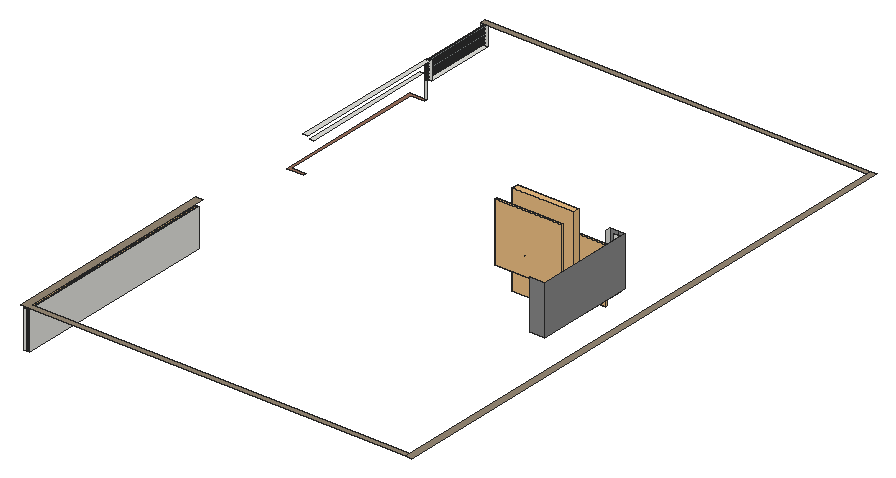
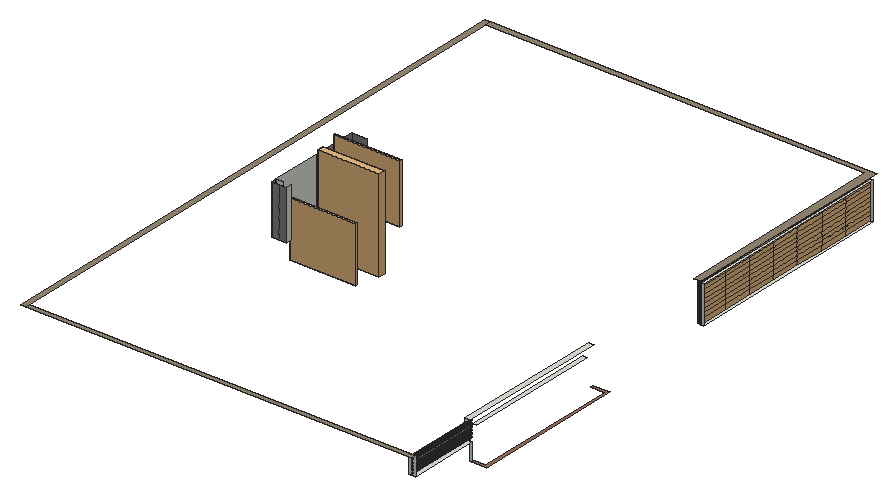
# SketchUp Ruby script. Lengths in inches.
U = 1.inch
M = Sketchup.active_model
def pt(a) = Geom::Point3d.new(a.map { |v| v * U })
def face(e, loops, mat)
  f = e.add_face(loops[0].map { |a| pt(a) })
  loops[1..].each { |l| e.add_face(l.map { |a| pt(a) }).erase! }
  f.material = f.back_material = mat if mat
  f
end
# faces: each face lists its corners as indices into pts; further lists are holes
def faces(e, pts, list, mat = nil) = list.each { |f| face(e, (f[0].is_a?(Array) ? f : [f]).map { |l| l.map { |i| pts[i] } }, mat) }
# xy, xz, yz: faces in a plane at the given z, y or x. An outline is a flat list of corners, or four numbers for a rectangle; further outlines are holes
def ring(l) = l.size == 4 ? [[l[0], l[1]], [l[2], l[1]], [l[2], l[3]], [l[0], l[3]]] : l.each_slice(2).to_a
def flat(e, list, mat, &to3) = list.each { |f| face(e, (f[0].is_a?(Array) ? f : [f]).map { |l| ring(l).map { |u, v| to3.(u, v) } }, mat) }
def xy(e, z, list, mat = nil) = flat(e, list, mat) { |x, y| [x, y, z] }
def xz(e, y, list, mat = nil) = flat(e, list, mat) { |x, z| [x, y, z] }
def yz(e, x, list, mat = nil) = flat(e, list, mat) { |y, z| [x, y, z] }
def lines(e, pts, list) = list.each { |a, b| e.add_line(pt(pts[a]), pt(pts[b])) }
# prism: a flat outline (further loops are holes) pulled along v
def prism(e, loops, v, mat = nil)
  f = face(e, loops, mat); d = Geom::Vector3d.new(v.map { |x| x * U })
  f.pushpull(f.normal.samedirection?(d) ? d.length : -d.length)
end
def box(e, o, s, mat = nil) = prism(e, [[o, [o[0] + s[0], o[1], o[2]], [o[0] + s[0], o[1] + s[1], o[2]], [o[0], o[1] + s[1], o[2]]]], [0, 0, s[2]], mat)
def at(x, y, z, deg = 0) = Geom::Transformation.translation(pt([x, y, z])) * Geom::Transformation.rotation(ORIGIN, Z_AXIS, deg.degrees)
def axes(o, x, y, z) = Geom::Transformation.new([*x, 0, *y, 0, *z, 0, *pt(o).to_a, 1])
def part(name) = M.definitions.add(name)
# library, detail: a bought-in or finely detailed component or shape, given as its bounding box
def library(name, o, s) = part(name).tap { |d| box(d.entities, o, s) }
def detail(e, o, s) = box(e.add_group.entities, o, s)
def put(e, d, t, mat = nil) = e.add_instance(d, t).tap { |i| i.material = mat if mat }
def group(e, t, mat = nil) = e.add_group.tap { |g| g.transformation = t; g.material = mat if mat }.entities
root = M.entities
M.materials.add("Bricks Weathered E01 100cm\#1").color = [154, 112, 93]
M.materials.add("Steel Blurry").color = [182, 192, 192]
M.materials.add("Wall Paint Bumpy 01 Gray 100cm").color = [135, 135, 135]
M.materials.add("Wall Paint Bumpy 01 Ochre 100cm").color = [152, 138, 118]
c1 = library("Decorative grille panel",[-1.9,0,0],[1.9,51.3,7.95])
c2 = library("Group\#6",[0,0,0],[112.45,3.15,94.27])
c3 = library("Group\#11",[0,0,0],[103.79,11.15,157.27])
c4 = part("Round post")
xy(c4.entities,0,[[1.13,0,0.86,0.03,0.6,0.12,0.37,0.27,0.1875,0.48,0.0625,0.72,0,0.99,0.01,1.27,0.08,1.53,0.22,1.77,0.42,1.97,0.65,2.11,0.92,2.19,1.2,2.19,1.46,2.14,1.71,2.01,1.92,1.83,2.07,1.6,2.17,1.34,2.19,1.07,2.15,0.8,2.04,0.54,1.875,0.32,1.66,0.15,1.4,0.04]])
xy(c4.entities,124.8,[[1.13,0,1.4,0.04,1.66,0.15,1.875,0.32,2.04,0.54,2.15,0.8,2.19,1.07,2.17,1.34,2.07,1.6,1.92,1.83,1.71,2.01,1.46,2.14,1.2,2.19,0.92,2.19,0.65,2.11,0.42,1.97,0.22,1.77,0.08,1.53,0.01,1.27,0,0.99,0.0625,0.72,0.1875,0.48,0.37,0.27,0.6,0.12,0.86,0.03]])
xz(c4.entities,2.19,[[0.92,0,1.2,124.8]],"Steel Blurry")
p = [[0.6,0.12,0],[0.86,0.03,0],[0.86,0.03,124.8],[0.6,0.12,124.8],[1.13,0,0],[1.13,0,124.8],
  [1.4,0.04,0],[1.4,0.04,124.8],[1.66,0.15,0],[1.66,0.15,124.8],[0.37,0.27,0],[0.37,0.27,124.8],
  [1.875,0.32,0],[1.875,0.32,124.8],[0.1875,0.48,0],[0.1875,0.48,124.8],[2.04,0.54,0],[2.04,0.54,124.8],
  [0.0625,0.72,0],[0.0625,0.72,124.8],[2.15,0.8,0],[2.15,0.8,124.8],[0,0.99,0],[0,0.99,124.8],
  [2.19,1.07,0],[2.19,1.07,124.8],[0.01,1.27,0],[0.01,1.27,124.8],[2.17,1.34,0],[2.17,1.34,124.8],
  [0.08,1.53,0],[0.08,1.53,124.8],[2.07,1.6,0],[2.07,1.6,124.8],[0.22,1.77,0],[0.22,1.77,124.8],
  [1.92,1.83,0],[1.92,1.83,124.8],[0.42,1.97,0],[0.42,1.97,124.8],[1.71,2.01,0],[1.71,2.01,124.8],
  [0.65,2.11,0],[0.65,2.11,124.8],[1.46,2.14,0],[1.46,2.14,124.8],[0.92,2.19,0],[0.92,2.19,124.8],
  [1.2,2.19,0],[1.2,2.19,124.8]]
faces(c4.entities,p,[[0,1,2,3],[1,4,5,2],[4,6,7,5],[6,8,9,7],[10,0,3,11],[8,12,13,9],[14,10,11,15],[12,16,17,13],
  [18,14,15,19],[16,20,21,17],[22,18,19,23],[20,24,25,21],[26,22,23,27],[24,28,29,25],[30,26,27,31],[28,32,33,29],
  [34,30,31,35],[32,36,37,33],[38,34,35,39],[36,40,41,37],[42,38,39,43],[40,44,45,41],[46,42,43,47],[44,48,49,45]],"Steel Blurry")
c5 = library("Group\#12",[0,0,0],[113.66,3.15,100.57])
xy(root,1.21,[[1729.02,411.88,1740.02,770.97]])
xy(root,6.3,[[2153.41,941.68,2153.67,941.68,2153.92,941.76,2154.15,941.89,2154.33,942.08,2154.45,942.31,2154.52,942.56,2154.51,942.82,2154.44,943.07,2154.31,943.3,2154.12,943.48,2153.89,943.6,2153.64,943.67,2153.38,943.66,2153.125,943.59,2152.9,943.46,2152.72,943.27,2152.59,943.04,2152.53,942.79,2152.53,942.53,2152.61,942.28,2152.74,942.05,2152.93,941.87,2153.16,941.74],[2153.49,979.17,2153.54,979.17,2153.56,979.18,2153.62,979.18,2153.64,979.1875,2153.66,979.19,2153.7,979.21,2153.72,979.21,2153.78,979.24,2153.79,979.25,2153.8125,979.26,2153.83,979.28,2153.84,979.29,2153.86,979.3,2153.875,979.32,2153.89,979.33,2153.9,979.35,2153.92,979.36,2153.95,979.42,2153.96,979.43,2154,979.51,2154,979.53,2154.01,979.55,2154.01,979.57,2154.02,979.59,2154.02,979.76,2154.01,979.78,2154.01,979.8,2154,979.82,2154,979.84,2153.96,979.92,2153.95,979.93,2153.93,979.97,2153.9,980,2153.89,980.02,2153.87,980.03,2153.86,980.05,2153.84,980.06,2153.81,980.09,2153.74,980.125,2153.72,980.14,2153.7,980.14,2153.66,980.16,2153.64,980.16,2153.62,980.17,2153.45,980.17,2153.43,980.16,2153.39,980.16,2153.33,980.13,2153.29,980.12,2153.25,980.1,2153.24,980.08,2153.2,980.06,2153.1875,980.04,2153.17,980.03,2153.14,980,2153.13,979.98,2153.12,979.97,2153.08,979.89,2153.06,979.86,2153.04,979.82,2153.04,979.8,2153.03,979.78,2153.03,979.71,2153.02,979.69,2153.02,979.65,2153.03,979.63,2153.03,979.59,2153.04,979.57,2153.04,979.55,2153.05,979.53,2153.05,979.51,2153.1,979.41,2153.11,979.4,2153.13,979.36,2153.15,979.35,2153.16,979.33,2153.18,979.32,2153.19,979.3,2153.21,979.29,2153.22,979.27,2153.28,979.24,2153.29,979.23,2153.3125,979.22,2153.33,979.21,2153.35,979.2,2153.37,979.2,2153.39,979.19,2153.41,979.1875,2153.43,979.18,2153.47,979.18]])
xy(root,9.5,[[1704.32,1001.07,1733.02,1001.07,1733.02,1005.17,1709.32,1005.17,1709.32,1257.65,1733.02,1257.65,1733.02,1262.67,1704.32,1262.67]],"Bricks Weathered E01 100cm\#1")
xy(root,12.6,[[2163.41,941.68,2163.67,941.68,2163.92,941.76,2164.15,941.89,2164.33,942.08,2164.45,942.31,2164.52,942.56,2164.51,942.82,2164.44,943.07,2164.31,943.3,2164.12,943.48,2163.89,943.6,2163.64,943.67,2163.38,943.66,2163.125,943.59,2162.9,943.46,2162.72,943.27,2162.59,943.04,2162.53,942.79,2162.53,942.53,2162.61,942.28,2162.74,942.05,2162.93,941.87,2163.16,941.74],[2163.49,979.17,2163.54,979.17,2163.56,979.18,2163.62,979.18,2163.64,979.1875,2163.66,979.19,2163.7,979.21,2163.72,979.21,2163.78,979.24,2163.79,979.25,2163.8125,979.26,2163.83,979.28,2163.84,979.29,2163.86,979.3,2163.875,979.32,2163.89,979.33,2163.9,979.35,2163.92,979.36,2163.95,979.42,2163.96,979.43,2164,979.51,2164,979.53,2164.01,979.55,2164.01,979.57,2164.02,979.59,2164.02,979.76,2164.01,979.78,2164.01,979.8,2164,979.82,2164,979.84,2163.96,979.92,2163.95,979.93,2163.93,979.97,2163.9,980,2163.89,980.02,2163.87,980.03,2163.86,980.05,2163.84,980.06,2163.81,980.09,2163.74,980.125,2163.72,980.14,2163.7,980.14,2163.66,980.16,2163.64,980.16,2163.62,980.17,2163.45,980.17,2163.43,980.16,2163.39,980.16,2163.33,980.13,2163.29,980.12,2163.25,980.1,2163.24,980.08,2163.2,980.06,2163.1875,980.04,2163.17,980.03,2163.14,980,2163.13,979.98,2163.12,979.97,2163.08,979.89,2163.06,979.86,2163.04,979.82,2163.04,979.8,2163.03,979.78,2163.03,979.71,2163.02,979.69,2163.02,979.65,2163.03,979.63,2163.03,979.59,2163.04,979.57,2163.04,979.55,2163.05,979.53,2163.05,979.51,2163.1,979.41,2163.11,979.4,2163.13,979.36,2163.15,979.35,2163.16,979.33,2163.18,979.32,2163.19,979.3,2163.21,979.29,2163.22,979.27,2163.28,979.24,2163.29,979.23,2163.3125,979.22,2163.33,979.21,2163.35,979.2,2163.37,979.2,2163.39,979.19,2163.41,979.1875,2163.43,979.18,2163.47,979.18]])
xy(root,18.9,[[2173.41,941.68,2173.67,941.68,2173.92,941.76,2174.15,941.89,2174.33,942.08,2174.45,942.31,2174.52,942.56,2174.51,942.82,2174.44,943.07,2174.31,943.3,2174.12,943.48,2173.89,943.6,2173.64,943.67,2173.38,943.66,2173.125,943.59,2172.9,943.46,2172.72,943.27,2172.59,943.04,2172.53,942.79,2172.53,942.53,2172.61,942.28,2172.74,942.05,2172.93,941.87,2173.16,941.74],[2173.49,979.17,2173.54,979.17,2173.56,979.18,2173.62,979.18,2173.64,979.1875,2173.66,979.19,2173.7,979.21,2173.72,979.21,2173.78,979.24,2173.79,979.25,2173.8125,979.26,2173.83,979.28,2173.84,979.29,2173.86,979.3,2173.875,979.32,2173.89,979.33,2173.9,979.35,2173.92,979.36,2173.95,979.42,2173.96,979.43,2174,979.51,2174,979.53,2174.01,979.55,2174.01,979.57,2174.02,979.59,2174.02,979.76,2174.01,979.78,2174.01,979.8,2174,979.82,2174,979.84,2173.96,979.92,2173.95,979.93,2173.93,979.97,2173.9,980,2173.89,980.02,2173.87,980.03,2173.86,980.05,2173.84,980.06,2173.81,980.09,2173.74,980.125,2173.72,980.14,2173.7,980.14,2173.66,980.16,2173.64,980.16,2173.62,980.17,2173.45,980.17,2173.43,980.16,2173.39,980.16,2173.33,980.13,2173.29,980.12,2173.25,980.1,2173.24,980.08,2173.2,980.06,2173.1875,980.04,2173.17,980.03,2173.14,980,2173.13,979.98,2173.12,979.97,2173.08,979.89,2173.06,979.86,2173.04,979.82,2173.04,979.8,2173.03,979.78,2173.03,979.71,2173.02,979.69,2173.02,979.65,2173.03,979.63,2173.03,979.59,2173.04,979.57,2173.04,979.55,2173.05,979.53,2173.05,979.51,2173.1,979.41,2173.11,979.4,2173.13,979.36,2173.15,979.35,2173.16,979.33,2173.18,979.32,2173.19,979.3,2173.21,979.29,2173.22,979.27,2173.28,979.24,2173.29,979.23,2173.3125,979.22,2173.33,979.21,2173.35,979.2,2173.37,979.2,2173.39,979.19,2173.41,979.1875,2173.43,979.18,2173.47,979.18]])
xy(root,25.2,[[2183.41,941.68,2183.67,941.68,2183.92,941.76,2184.15,941.89,2184.33,942.08,2184.45,942.31,2184.52,942.56,2184.51,942.82,2184.44,943.07,2184.31,943.3,2184.12,943.48,2183.89,943.6,2183.64,943.67,2183.38,943.66,2183.125,943.59,2182.9,943.46,2182.72,943.27,2182.59,943.04,2182.53,942.79,2182.53,942.53,2182.61,942.28,2182.74,942.05,2182.93,941.87,2183.16,941.74],[2183.49,979.17,2183.54,979.17,2183.56,979.18,2183.62,979.18,2183.64,979.1875,2183.66,979.19,2183.7,979.21,2183.72,979.21,2183.78,979.24,2183.79,979.25,2183.8125,979.26,2183.83,979.28,2183.84,979.29,2183.86,979.3,2183.875,979.32,2183.89,979.33,2183.9,979.35,2183.92,979.36,2183.95,979.42,2183.96,979.43,2184,979.51,2184,979.53,2184.01,979.55,2184.01,979.57,2184.02,979.59,2184.02,979.76,2184.01,979.78,2184.01,979.8,2184,979.82,2184,979.84,2183.96,979.92,2183.95,979.93,2183.93,979.97,2183.9,980,2183.89,980.02,2183.87,980.03,2183.86,980.05,2183.84,980.06,2183.81,980.09,2183.74,980.125,2183.72,980.14,2183.7,980.14,2183.66,980.16,2183.64,980.16,2183.62,980.17,2183.45,980.17,2183.43,980.16,2183.39,980.16,2183.33,980.13,2183.29,980.12,2183.25,980.1,2183.24,980.08,2183.2,980.06,2183.1875,980.04,2183.17,980.03,2183.14,980,2183.13,979.98,2183.12,979.97,2183.08,979.89,2183.06,979.86,2183.04,979.82,2183.04,979.8,2183.03,979.78,2183.03,979.71,2183.02,979.69,2183.02,979.65,2183.03,979.63,2183.03,979.59,2183.04,979.57,2183.04,979.55,2183.05,979.53,2183.05,979.51,2183.1,979.41,2183.11,979.4,2183.13,979.36,2183.15,979.35,2183.16,979.33,2183.18,979.32,2183.19,979.3,2183.21,979.29,2183.22,979.27,2183.28,979.24,2183.29,979.23,2183.3125,979.22,2183.33,979.21,2183.35,979.2,2183.37,979.2,2183.39,979.19,2183.41,979.1875,2183.43,979.18,2183.47,979.18]])
xy(root,31.5,[[2193.49,979.17,2193.54,979.17,2193.56,979.18,2193.62,979.18,2193.64,979.1875,2193.66,979.19,2193.7,979.21,2193.72,979.21,2193.78,979.24,2193.79,979.25,2193.8125,979.26,2193.83,979.28,2193.84,979.29,2193.86,979.3,2193.875,979.32,2193.89,979.33,2193.9,979.35,2193.92,979.36,2193.95,979.42,2193.96,979.43,2194,979.51,2194,979.53,2194.01,979.55,2194.01,979.57,2194.02,979.59,2194.02,979.76,2194.01,979.78,2194.01,979.8,2194,979.82,2194,979.84,2193.96,979.92,2193.95,979.93,2193.93,979.97,2193.9,980,2193.89,980.02,2193.87,980.03,2193.86,980.05,2193.84,980.06,2193.81,980.09,2193.74,980.125,2193.72,980.14,2193.7,980.14,2193.66,980.16,2193.64,980.16,2193.62,980.17,2193.45,980.17,2193.43,980.16,2193.39,980.16,2193.33,980.13,2193.29,980.12,2193.25,980.1,2193.24,980.08,2193.2,980.06,2193.1875,980.04,2193.17,980.03,2193.14,980,2193.13,979.98,2193.12,979.97,2193.08,979.89,2193.06,979.86,2193.04,979.82,2193.04,979.8,2193.03,979.78,2193.03,979.71,2193.02,979.69,2193.02,979.65,2193.03,979.63,2193.03,979.59,2193.04,979.57,2193.04,979.55,2193.05,979.53,2193.05,979.51,2193.1,979.41,2193.11,979.4,2193.13,979.36,2193.15,979.35,2193.16,979.33,2193.18,979.32,2193.19,979.3,2193.21,979.29,2193.22,979.27,2193.28,979.24,2193.29,979.23,2193.3125,979.22,2193.33,979.21,2193.35,979.2,2193.37,979.2,2193.39,979.19,2193.41,979.1875,2193.43,979.18,2193.47,979.18]])
xy(root,37.8,[[2203.41,941.68,2203.67,941.68,2203.92,941.76,2204.15,941.89,2204.33,942.08,2204.45,942.31,2204.52,942.56,2204.51,942.82,2204.44,943.07,2204.31,943.3,2204.12,943.48,2203.89,943.6,2203.64,943.67,2203.38,943.66,2203.125,943.59,2202.9,943.46,2202.72,943.27,2202.59,943.04,2202.53,942.79,2202.53,942.53,2202.61,942.28,2202.74,942.05,2202.93,941.87,2203.16,941.74],[2203.56,979.17,2203.61,979.17,2203.63,979.18,2203.69,979.18,2203.71,979.1875,2203.73,979.19,2203.77,979.21,2203.79,979.21,2203.85,979.24,2203.86,979.25,2203.88,979.26,2203.91,979.29,2203.93,979.3,2203.96,979.33,2203.97,979.35,2203.99,979.36,2204.02,979.42,2204.03,979.43,2204.07,979.51,2204.07,979.53,2204.08,979.55,2204.08,979.57,2204.09,979.59,2204.09,979.76,2204.08,979.78,2204.08,979.8,2204.07,979.82,2204.07,979.84,2204.03,979.92,2204.02,979.93,2203.99,979.99,2203.97,980,2203.96,980.02,2203.94,980.03,2203.93,980.05,2203.91,980.06,2203.88,980.09,2203.81,980.125,2203.79,980.14,2203.77,980.14,2203.73,980.16,2203.71,980.16,2203.6875,980.17,2203.52,980.17,2203.5,980.16,2203.46,980.16,2203.4375,980.15,2203.42,980.14,2203.4,980.13,2203.36,980.12,2203.34,980.11,2203.31,980.08,2203.27,980.06,2203.26,980.04,2203.24,980.03,2203.21,980,2203.2,979.98,2203.1875,979.97,2203.18,979.95,2203.15,979.89,2203.13,979.86,2203.12,979.84,2203.12,979.82,2203.11,979.8,2203.11,979.78,2203.1,979.76,2203.1,979.71,2203.09,979.69,2203.09,979.65,2203.1,979.63,2203.1,979.59,2203.11,979.57,2203.11,979.55,2203.12,979.53,2203.12,979.51,2203.17,979.41,2203.18,979.4,2203.2,979.36,2203.22,979.35,2203.23,979.33,2203.25,979.32,2203.26,979.3,2203.28,979.29,2203.29,979.27,2203.35,979.24,2203.36,979.23,2203.42,979.2,2203.44,979.2,2203.46,979.19,2203.48,979.1875,2203.5,979.18,2203.54,979.18]])
xy(root,40.2,[[1729.02,1262.67,1741.02,1382.67]])
xy(root,44.1,[[2213.41,941.68,2213.67,941.68,2213.92,941.76,2214.15,941.89,2214.33,942.08,2214.45,942.31,2214.52,942.56,2214.51,942.82,2214.44,943.07,2214.31,943.3,2214.12,943.48,2213.89,943.6,2213.64,943.67,2213.38,943.66,2213.125,943.59,2212.9,943.46,2212.72,943.27,2212.59,943.04,2212.53,942.79,2212.53,942.53,2212.61,942.28,2212.74,942.05,2212.93,941.87,2213.16,941.74],[2213.56,979.17,2213.61,979.17,2213.63,979.18,2213.69,979.18,2213.71,979.1875,2213.73,979.19,2213.77,979.21,2213.79,979.21,2213.85,979.24,2213.86,979.25,2213.88,979.26,2213.91,979.29,2213.93,979.3,2213.96,979.33,2213.97,979.35,2213.99,979.36,2214.02,979.42,2214.03,979.43,2214.07,979.51,2214.07,979.53,2214.08,979.55,2214.08,979.57,2214.09,979.59,2214.09,979.76,2214.08,979.78,2214.08,979.8,2214.07,979.82,2214.07,979.84,2214.03,979.92,2214.02,979.93,2213.99,979.99,2213.97,980,2213.96,980.02,2213.94,980.03,2213.93,980.05,2213.91,980.06,2213.88,980.09,2213.81,980.125,2213.79,980.14,2213.77,980.14,2213.73,980.16,2213.71,980.16,2213.6875,980.17,2213.52,980.17,2213.5,980.16,2213.46,980.16,2213.4375,980.15,2213.42,980.14,2213.4,980.13,2213.36,980.12,2213.34,980.11,2213.31,980.08,2213.27,980.06,2213.26,980.04,2213.24,980.03,2213.21,980,2213.2,979.98,2213.1875,979.97,2213.18,979.95,2213.15,979.89,2213.13,979.86,2213.12,979.84,2213.12,979.82,2213.11,979.8,2213.11,979.78,2213.1,979.76,2213.1,979.71,2213.09,979.69,2213.09,979.65,2213.1,979.63,2213.1,979.59,2213.11,979.57,2213.11,979.55,2213.12,979.53,2213.12,979.51,2213.17,979.41,2213.18,979.4,2213.2,979.36,2213.22,979.35,2213.23,979.33,2213.25,979.32,2213.26,979.3,2213.28,979.29,2213.29,979.27,2213.35,979.24,2213.36,979.23,2213.42,979.2,2213.44,979.2,2213.46,979.19,2213.48,979.1875,2213.5,979.18,2213.54,979.18]])
xy(root,50.4,[[2223.56,979.17,2223.61,979.17,2223.63,979.18,2223.69,979.18,2223.71,979.1875,2223.73,979.19,2223.77,979.21,2223.79,979.21,2223.85,979.24,2223.86,979.25,2223.88,979.26,2223.91,979.29,2223.93,979.3,2223.96,979.33,2223.97,979.35,2223.99,979.36,2224.02,979.42,2224.03,979.43,2224.07,979.51,2224.07,979.53,2224.08,979.55,2224.08,979.57,2224.09,979.59,2224.09,979.76,2224.08,979.78,2224.08,979.8,2224.07,979.82,2224.07,979.84,2224.03,979.92,2224.02,979.93,2223.99,979.99,2223.97,980,2223.96,980.02,2223.94,980.03,2223.93,980.05,2223.91,980.06,2223.88,980.09,2223.81,980.125,2223.79,980.14,2223.77,980.14,2223.73,980.16,2223.71,980.16,2223.6875,980.17,2223.52,980.17,2223.5,980.16,2223.46,980.16,2223.4375,980.15,2223.42,980.14,2223.4,980.13,2223.36,980.12,2223.34,980.11,2223.31,980.08,2223.27,980.06,2223.26,980.04,2223.24,980.03,2223.21,980,2223.2,979.98,2223.1875,979.97,2223.18,979.95,2223.15,979.89,2223.13,979.86,2223.12,979.84,2223.12,979.82,2223.11,979.8,2223.11,979.78,2223.1,979.76,2223.1,979.71,2223.09,979.69,2223.09,979.65,2223.1,979.63,2223.1,979.59,2223.11,979.57,2223.11,979.55,2223.12,979.53,2223.12,979.51,2223.17,979.41,2223.18,979.4,2223.2,979.36,2223.22,979.35,2223.23,979.33,2223.25,979.32,2223.26,979.3,2223.28,979.29,2223.29,979.27,2223.35,979.24,2223.36,979.23,2223.42,979.2,2223.44,979.2,2223.46,979.19,2223.48,979.1875,2223.5,979.18,2223.54,979.18]])
xy(root,56.7,[[2233.49,979.17,2233.54,979.17,2233.56,979.18,2233.62,979.18,2233.64,979.1875,2233.66,979.19,2233.7,979.21,2233.72,979.21,2233.78,979.24,2233.79,979.25,2233.8125,979.26,2233.83,979.28,2233.84,979.29,2233.86,979.3,2233.875,979.32,2233.89,979.33,2233.9,979.35,2233.92,979.36,2233.95,979.42,2233.96,979.43,2234,979.51,2234,979.53,2234.01,979.55,2234.01,979.57,2234.02,979.59,2234.02,979.76,2234.01,979.78,2234.01,979.8,2234,979.82,2234,979.84,2233.96,979.92,2233.95,979.93,2233.93,979.97,2233.9,980,2233.89,980.02,2233.87,980.03,2233.86,980.05,2233.84,980.06,2233.81,980.09,2233.74,980.125,2233.72,980.14,2233.7,980.14,2233.66,980.16,2233.64,980.16,2233.62,980.17,2233.45,980.17,2233.43,980.16,2233.39,980.16,2233.33,980.13,2233.29,980.12,2233.25,980.1,2233.24,980.08,2233.2,980.06,2233.1875,980.04,2233.17,980.03,2233.14,980,2233.13,979.98,2233.12,979.97,2233.08,979.89,2233.06,979.86,2233.04,979.82,2233.04,979.8,2233.03,979.78,2233.03,979.71,2233.02,979.69,2233.02,979.65,2233.03,979.63,2233.03,979.59,2233.04,979.57,2233.04,979.55,2233.05,979.53,2233.05,979.51,2233.1,979.41,2233.11,979.4,2233.13,979.36,2233.15,979.35,2233.16,979.33,2233.18,979.32,2233.19,979.3,2233.21,979.29,2233.22,979.27,2233.28,979.24,2233.29,979.23,2233.3125,979.22,2233.33,979.21,2233.35,979.2,2233.37,979.2,2233.39,979.19,2233.41,979.1875,2233.43,979.18,2233.47,979.18]])
xy(root,58.01,[[1733.02,1014.17,1740.02,1248.68]])
xy(root,64.79,[[1729.02,411.88,1740.02,770.97]])
xy(root,72,[[1733.02,1000.17,1741.02,1262.67]])
xy(root,72,[[1729.02,404.67,2384.52,404.67,2384.52,413.67,1741.02,413.67,1741.02,778.17,1729.02,778.17],[2384.52,404.67,2393.52,1391.67],[1729.02,1382.67,2384.52,1391.67]],"Wall Paint Bumpy 01 Ochre 100cm")
xy(root,94.5,[[2193.41,896.68,2193.67,896.68,2193.92,896.76,2194.15,896.89,2194.33,897.08,2194.45,897.31,2194.52,897.56,2194.51,897.82,2194.44,898.07,2194.31,898.3,2194.12,898.48,2193.89,898.6,2193.64,898.67,2193.38,898.66,2193.125,898.59,2192.9,898.46,2192.72,898.27,2192.59,898.04,2192.53,897.79,2192.53,897.53,2192.61,897.28,2192.74,897.05,2192.93,896.87,2193.16,896.74]])
xy(root,100.8,[[2183.41,896.68,2183.67,896.68,2183.92,896.76,2184.15,896.89,2184.33,897.08,2184.45,897.31,2184.52,897.56,2184.51,897.82,2184.44,898.07,2184.31,898.3,2184.12,898.48,2183.89,898.6,2183.64,898.67,2183.38,898.66,2183.125,898.59,2182.9,898.46,2182.72,898.27,2182.59,898.04,2182.53,897.79,2182.53,897.53,2182.61,897.28,2182.74,897.05,2182.93,896.87,2183.16,896.74],[2183.41,933.68,2183.67,933.68,2183.92,933.76,2184.15,933.89,2184.33,934.08,2184.45,934.31,2184.52,934.56,2184.51,934.82,2184.44,935.07,2184.31,935.3,2184.12,935.48,2183.89,935.6,2183.64,935.67,2183.38,935.66,2183.125,935.59,2182.9,935.46,2182.72,935.27,2182.59,935.04,2182.53,934.79,2182.53,934.53,2182.61,934.28,2182.74,934.05,2182.93,933.87,2183.16,933.74]])
xy(root,107.1,[[2173.65,896.68,2173.91,896.68,2174.17,896.76,2174.39,896.89,2174.57,897.08,2174.7,897.31,2174.76,897.56,2174.76,897.82,2174.6875,898.07,2174.55,898.3,2174.36,898.48,2174.14,898.6,2173.88,898.67,2173.62,898.66,2173.37,898.59,2173.15,898.46,2172.97,898.27,2172.84,898.04,2172.77,897.79,2172.78,897.53,2172.85,897.28,2172.98,897.05,2173.17,896.87,2173.4,896.74],[2173.41,933.68,2173.67,933.68,2173.92,933.76,2174.15,933.89,2174.33,934.08,2174.45,934.31,2174.52,934.56,2174.51,934.82,2174.44,935.07,2174.31,935.3,2174.12,935.48,2173.89,935.6,2173.64,935.67,2173.38,935.66,2173.125,935.59,2172.9,935.46,2172.72,935.27,2172.59,935.04,2172.53,934.79,2172.53,934.53,2172.61,934.28,2172.74,934.05,2172.93,933.87,2173.16,933.74]])
xy(root,113.4,[[2163.65,896.89,2163.91,896.9,2164.17,896.97,2164.39,897.1,2164.57,897.29,2164.7,897.52,2164.76,897.77,2164.76,898.03,2164.6875,898.28,2164.55,898.51,2164.36,898.69,2164.14,898.82,2163.88,898.88,2163.62,898.875,2163.37,898.81,2163.15,898.67,2162.97,898.48,2162.84,898.26,2162.77,898,2162.78,897.74,2162.85,897.49,2162.98,897.27,2163.17,897.08,2163.4,896.96],[2163.41,933.68,2163.67,933.68,2163.92,933.76,2164.15,933.89,2164.33,934.08,2164.45,934.31,2164.52,934.56,2164.51,934.82,2164.44,935.07,2164.31,935.3,2164.12,935.48,2163.89,935.6,2163.64,935.67,2163.38,935.66,2163.125,935.59,2162.9,935.46,2162.72,935.27,2162.59,935.04,2162.53,934.79,2162.53,934.53,2162.61,934.28,2162.74,934.05,2162.93,933.87,2163.16,933.74]])
xz(root,411.88,[[1729.02,1.21,1740.02,64.79]])
xz(root,770.97,[[1729.02,1.21,1740.02,64.79]])
xz(root,819.67,[[2262.52,36,2288.52,120]],"Wall Paint Bumpy 01 Gray 100cm")
xz(root,980.67,[[2276.52,36,2287.52,120]])
xz(root,989.67,[[2262.52,36,2276.52,120],[2276.52,36,2288.52,120]],"Wall Paint Bumpy 01 Gray 100cm")
xz(root,1262.67,[[1729.02,9.5,1733.02,40.2],[1733.02,40.2,1741.02,72]])
xz(root,1382.67,[[1729.02,40.2,1741.02,72]])
yz(root,1740.02,[[411.88,1.21,770.97,64.79]])
yz(root,2287.52,[[896.67,36,980.67,120]])
yz(root,2288.52,[[819.67,36,989.67,120]],"Wall Paint Bumpy 01 Gray 100cm")
p = [[2262.52,980.67,36],[2262.52,980.67,120],[2262.33,989.53,120],[2262.33,989.53,36],[2262.52,887.67,36],[2262.52,819.67,36]]
faces(root,p,[[0,1,2,3]])
lines(root,p,[[4,5]])
g1 = group(root,at(1736.42,411.88,1.21))
put(g1,c1,axes([0,0,0],[1,0,0],[0,1,0],[0,0,0.88889]))
put(g1,c1,axes([0,51.3,0],[1,0,0],[0,1,0],[0,0,0.88889]))
put(g1,c1,axes([0,102.6,0],[1,0,0],[0,1,0],[0,0,0.88889]))
put(g1,c1,axes([0,153.89,0],[1,0,0],[0,1,0],[0,0,0.88889]))
put(g1,c1,axes([0,205.19,0],[1,0,0],[0,1,0],[0,0,0.88889]))
put(g1,c1,axes([0,256.49,0],[1,0,0],[0,1,0],[0,0,0.88889]))
put(g1,c1,axes([0,307.79,0],[1,0,0],[0,1,0],[0,0,0.88889]))
put(g1,c1,axes([0,102.6,7.07],[1,0,0],[0,1,0],[0,0,0.88889]))
put(g1,c1,axes([0,205.19,7.07],[1,0,0],[0,1,0],[0,0,0.88889]))
put(g1,c1,axes([0,256.49,7.07],[1,0,0],[0,1,0],[0,0,0.88889]))
put(g1,c1,axes([0,0,7.07],[1,0,0],[0,1,0],[0,0,0.88889]))
put(g1,c1,axes([0,51.3,7.07],[1,0,0],[0,1,0],[0,0,0.88889]))
put(g1,c1,axes([0,153.89,7.07],[1,0,0],[0,1,0],[0,0,0.88889]))
put(g1,c1,axes([0,307.79,7.07],[1,0,0],[0,1,0],[0,0,0.88889]))
put(g1,c1,axes([0,102.6,14.13],[1,0,0],[0,1,0],[0,0,0.88889]))
put(g1,c1,axes([0,205.19,14.13],[1,0,0],[0,1,0],[0,0,0.88889]))
put(g1,c1,axes([0,256.49,14.13],[1,0,0],[0,1,0],[0,0,0.88889]))
put(g1,c1,axes([0,0,14.13],[1,0,0],[0,1,0],[0,0,0.88889]))
put(g1,c1,axes([0,51.3,14.13],[1,0,0],[0,1,0],[0,0,0.88889]))
put(g1,c1,axes([0,153.89,14.13],[1,0,0],[0,1,0],[0,0,0.88889]))
put(g1,c1,axes([0,307.79,14.13],[1,0,0],[0,1,0],[0,0,0.88889]))
put(g1,c1,axes([0,102.6,21.2],[1,0,0],[0,1,0],[0,0,0.88889]))
put(g1,c1,axes([0,205.19,21.2],[1,0,0],[0,1,0],[0,0,0.88889]))
put(g1,c1,axes([0,256.49,21.2],[1,0,0],[0,1,0],[0,0,0.88889]))
put(g1,c1,axes([0,0,21.2],[1,0,0],[0,1,0],[0,0,0.88889]))
put(g1,c1,axes([0,51.3,21.2],[1,0,0],[0,1,0],[0,0,0.88889]))
put(g1,c1,axes([0,153.89,21.2],[1,0,0],[0,1,0],[0,0,0.88889]))
put(g1,c1,axes([0,307.79,21.2],[1,0,0],[0,1,0],[0,0,0.88889]))
put(g1,c1,axes([0,102.6,28.26],[1,0,0],[0,1,0],[0,0,0.88889]))
put(g1,c1,axes([0,205.19,28.26],[1,0,0],[0,1,0],[0,0,0.88889]))
put(g1,c1,axes([0,256.49,28.26],[1,0,0],[0,1,0],[0,0,0.88889]))
put(g1,c1,axes([0,0,28.26],[1,0,0],[0,1,0],[0,0,0.88889]))
put(g1,c1,axes([0,51.3,28.26],[1,0,0],[0,1,0],[0,0,0.88889]))
put(g1,c1,axes([0,153.89,28.26],[1,0,0],[0,1,0],[0,0,0.88889]))
put(g1,c1,axes([0,307.79,28.26],[1,0,0],[0,1,0],[0,0,0.88889]))
put(g1,c1,axes([0,102.6,35.33],[1,0,0],[0,1,0],[0,0,0.88889]))
put(g1,c1,axes([0,205.19,35.33],[1,0,0],[0,1,0],[0,0,0.88889]))
put(g1,c1,axes([0,256.49,35.33],[1,0,0],[0,1,0],[0,0,0.88889]))
put(g1,c1,axes([0,0,35.33],[1,0,0],[0,1,0],[0,0,0.88889]))
put(g1,c1,axes([0,51.3,35.33],[1,0,0],[0,1,0],[0,0,0.88889]))
put(g1,c1,axes([0,153.89,35.33],[1,0,0],[0,1,0],[0,0,0.88889]))
put(g1,c1,axes([0,307.79,35.33],[1,0,0],[0,1,0],[0,0,0.88889]))
put(g1,c1,axes([0,102.6,42.39],[1,0,0],[0,1,0],[0,0,0.88889]))
put(g1,c1,axes([0,205.19,42.39],[1,0,0],[0,1,0],[0,0,0.88889]))
put(g1,c1,axes([0,256.49,42.39],[1,0,0],[0,1,0],[0,0,0.88889]))
put(g1,c1,axes([0,0,42.39],[1,0,0],[0,1,0],[0,0,0.88889]))
put(g1,c1,axes([0,51.3,42.39],[1,0,0],[0,1,0],[0,0,0.88889]))
put(g1,c1,axes([0,153.89,42.39],[1,0,0],[0,1,0],[0,0,0.88889]))
put(g1,c1,axes([0,307.79,42.39],[1,0,0],[0,1,0],[0,0,0.88889]))
put(g1,c1,axes([0,102.6,49.46],[1,0,0],[0,1,0],[0,0,0.88889]))
put(g1,c1,axes([0,205.19,49.46],[1,0,0],[0,1,0],[0,0,0.88889]))
put(g1,c1,axes([0,256.49,49.46],[1,0,0],[0,1,0],[0,0,0.88889]))
put(g1,c1,axes([0,0,49.46],[1,0,0],[0,1,0],[0,0,0.88889]))
put(g1,c1,axes([0,51.3,49.46],[1,0,0],[0,1,0],[0,0,0.88889]))
put(g1,c1,axes([0,153.89,49.46],[1,0,0],[0,1,0],[0,0,0.88889]))
put(g1,c1,axes([0,307.79,49.46],[1,0,0],[0,1,0],[0,0,0.88889]))
put(g1,c1,axes([0,102.6,56.52],[1,0,0],[0,1,0],[0,0,0.88889]))
put(g1,c1,axes([0,205.19,56.52],[1,0,0],[0,1,0],[0,0,0.88889]))
put(g1,c1,axes([0,256.49,56.52],[1,0,0],[0,1,0],[0,0,0.88889]))
put(g1,c1,axes([0,0,56.52],[1,0,0],[0,1,0],[0,0,0.88889]))
put(g1,c1,axes([0,51.3,56.52],[1,0,0],[0,1,0],[0,0,0.88889]))
put(g1,c1,axes([0,153.89,56.52],[1,0,0],[0,1,0],[0,0,0.88889]))
put(g1,c1,axes([0,307.79,56.52],[1,0,0],[0,1,0],[0,0,0.88889]))
put(root,c2,at(2152.15,978.1,6.3))
put(root,c3,at(2141.95,933.1,6.3))
put(root,c4,axes([1733.21,1382.67,42.32],[1,0,0],[0,0,1],[0,-1,0]))
put(root,c4,axes([1733.21,1382.67,47.54],[1,0,0],[0,0,1],[0,-1,0]))
put(root,c4,axes([1733.21,1382.67,52.76],[1,0,0],[0,0,1],[0,-1,0]))
put(root,c4,axes([1733.21,1382.67,57.98],[1,0,0],[0,0,1],[0,-1,0]))
put(root,c5,at(2141.95,896.1,63))
put(root,c4,axes([1733.21,1382.67,63.2],[1,0,0],[0,0,1],[0,-1,0]))
put(root,c4,axes([1733.21,1382.67,68.42],[1,0,0],[0,0,1],[0,-1,0]))
